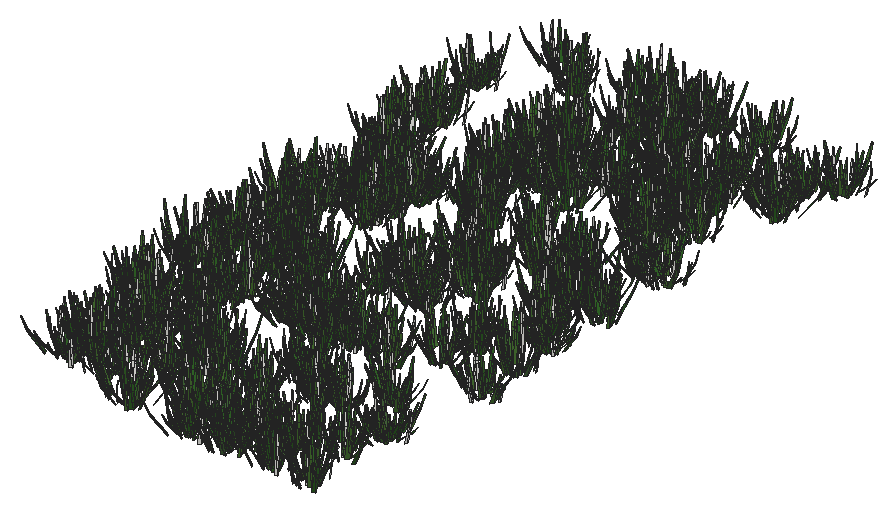
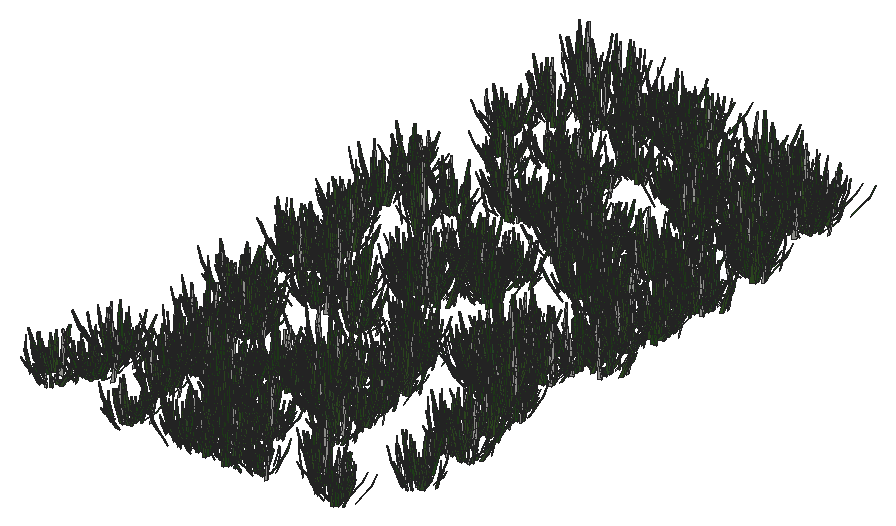
# SketchUp Ruby script. Lengths in inches.
U = 1.inch
M = Sketchup.active_model
def pt(a) = Geom::Point3d.new(a.map { |v| v * U })
def face(e, loops, mat)
  f = e.add_face(loops[0].map { |a| pt(a) })
  loops[1..].each { |l| e.add_face(l.map { |a| pt(a) }).erase! }
  f.material = f.back_material = mat if mat
  f
end
# faces: each face lists its corners as indices into pts; further lists are holes
def faces(e, pts, list, mat = nil) = list.each { |f| face(e, (f[0].is_a?(Array) ? f : [f]).map { |l| l.map { |i| pts[i] } }, mat) }
# xy, xz, yz: faces in a plane at the given z, y or x. An outline is a flat list of corners, or four numbers for a rectangle; further outlines are holes
def ring(l) = l.size == 4 ? [[l[0], l[1]], [l[2], l[1]], [l[2], l[3]], [l[0], l[3]]] : l.each_slice(2).to_a
def flat(e, list, mat, &to3) = list.each { |f| face(e, (f[0].is_a?(Array) ? f : [f]).map { |l| ring(l).map { |u, v| to3.(u, v) } }, mat) }
def xy(e, z, list, mat = nil) = flat(e, list, mat) { |x, y| [x, y, z] }
def xz(e, y, list, mat = nil) = flat(e, list, mat) { |x, z| [x, y, z] }
def yz(e, x, list, mat = nil) = flat(e, list, mat) { |y, z| [x, y, z] }
def lines(e, pts, list) = list.each { |a, b| e.add_line(pt(pts[a]), pt(pts[b])) }
# prism: a flat outline (further loops are holes) pulled along v
def prism(e, loops, v, mat = nil)
  f = face(e, loops, mat); d = Geom::Vector3d.new(v.map { |x| x * U })
  f.pushpull(f.normal.samedirection?(d) ? d.length : -d.length)
end
def box(e, o, s, mat = nil) = prism(e, [[o, [o[0] + s[0], o[1], o[2]], [o[0] + s[0], o[1] + s[1], o[2]], [o[0], o[1] + s[1], o[2]]]], [0, 0, s[2]], mat)
def at(x, y, z, deg = 0) = Geom::Transformation.translation(pt([x, y, z])) * Geom::Transformation.rotation(ORIGIN, Z_AXIS, deg.degrees)
def axes(o, x, y, z) = Geom::Transformation.new([*x, 0, *y, 0, *z, 0, *pt(o).to_a, 1])
def part(name) = M.definitions.add(name)
# library, detail: a bought-in or finely detailed component or shape, given as its bounding box
def library(name, o, s) = part(name).tap { |d| box(d.entities, o, s) }
def detail(e, o, s) = box(e.add_group.entities, o, s)
def put(e, d, t, mat = nil) = e.add_instance(d, t).tap { |i| i.material = mat if mat }
def group(e, t, mat = nil) = e.add_group.tap { |g| g.transformation = t; g.material = mat if mat }.entities
root = M.entities
M.materials.add("Material1").color = [58, 110, 58]
M.materials.add("Material10").color = [48, 100, 38]
M.materials.add("Material3").color = [68, 110, 58]
M.materials.add("Material4").color = [48, 90, 38]
M.materials.add("Material5").color = [68, 110, 48]
M.materials.add("Material6").color = [48, 90, 48]
M.materials.add("Material8").color = [58, 90, 38]
M.materials.add("Material9").color = [68, 100, 58]
c1 = part("grass00")
p = [[-0.6875,0.15,0],[-0.56,0.08,5.52],[-0.04,0.03,2.76],[0.48,-0.02,0],[0.35,-0.02,5.52],[-0.1,-0.14,5.52],
  [-0.12,0.65,8.37],[-0.42,0.65,8.37]]
faces(c1.entities,p,[[0,1,2,3],[3,2,4],[1,5,2],[5,4,2],[1,6,5],[4,5,6],[7,6,1]])
c2 = part("Group16\#1")
put(c2.entities,c1,axes([1.44,-0.61,-0.01],[0.05352,0.12609,0],[-0.10704,0.04543,0.07239],[0.06664,-0.02828,0.11628]),"Material6")
put(c2.entities,c1,axes([0.76,-0.15,-0.01],[0.04676,0.24062,0],[-0.23162,0.04501,0.06642],[0.0652,-0.01267,0.23595]),"Material3")
put(c2.entities,c1,axes([0.79,0.01,-0.01],[-0.00606,0.34651,0],[-0.34381,-0.00602,0.0432],[0.04319,0.00076,0.34386]))
put(c2.entities,c1,axes([1,0.23,-0.01],[-0.07192,0.31144,0],[-0.28722,-0.06632,0.1236],[0.12043,0.02781,0.29478]),"Material5")
put(c2.entities,c1,axes([1.66,0.77,-0.01],[-0.13828,0.29651,0],[-0.21551,-0.1005,0.22471],[0.20365,0.09498,0.23779]),"Material10")
put(c2.entities,c1,axes([0.6875,0.52,-0.01],[-0.18126,0.24051,0],[-0.22746,-0.17142,0.09788],[0.07817,0.05891,0.28481]),"Material5")
put(c2.entities,c1,axes([0.68,0.78,-0.01],[-0.215,0.18688,0],[-0.12385,-0.14248,0.21334],[0.13995,0.16101,0.18878]),"Material3")
put(c2.entities,c1,axes([0.56,1,-0.01],[-0.13756,0.07624,0],[-0.06159,-0.11112,0.0927],[0.04494,0.08108,0.12705]),"Material5")
put(c2.entities,c1,axes([0.2,0.64,-0.01],[-0.23729,0.07254,0],[-0.05711,-0.18681,0.153],[0.04473,0.14632,0.19535]),"Material10")
put(c2.entities,c1,axes([0.0625,0.72,-0.01],[-0.28874,0.02525,0],[-0.02179,-0.24916,0.14647],[0.01276,0.14591,0.25012]),"Material3")
put(c2.entities,c1,axes([-0.08,0.62,-0.01],[-0.34089,-0.04187,0],[0.03255,-0.26504,0.216],[-0.02633,0.21439,0.26703]),"Material10")
put(c2.entities,c1,axes([-0.34,0.98,-0.01],[-0.14314,-0.0493,0],[0.04397,-0.12769,0.06843],[-0.02228,0.0647,0.13505]),"Material10")
put(c2.entities,c1,axes([-0.87,1.45,-0.01],[-0.23488,-0.14114,0],[0.13761,-0.22901,0.06087],[-0.03135,0.05217,0.26717]))
put(c2.entities,c1,axes([-0.72,0.77,-0.01],[-0.14208,-0.13251,0],[0.07209,-0.0773,0.16301],[-0.11118,0.11922,0.1057]),"Material10")
put(c2.entities,c1,axes([-0.62,0.43,-0.01],[-0.14845,-0.21203,0],[0.18654,-0.13061,0.12304],[-0.10079,0.07057,0.22772]),"Material3")
put(c2.entities,c1,axes([-0.68,0.29,-0.01],[-0.13639,-0.32136,0],[0.31723,-0.13464,0.05579],[-0.05136,0.0218,0.34462]),"Material4")
put(c2.entities,c1,axes([-0.64,0.125,-0.01],[-0.0458,-0.23569,0],[0.22124,-0.043,0.08276],[-0.08124,0.01579,0.22538]),"Material1")
put(c2.entities,c1,axes([-1.6,-0.03,-0.01],[0.00576,-0.32897,0],[0.27526,0.00482,0.18018],[-0.18015,-0.00315,0.2753]),"Material5")
put(c2.entities,c1,axes([-1.36,-0.31,-0.01],[0.05718,-0.24765,0],[0.18172,0.04196,0.17267],[-0.16825,-0.03885,0.1865]),"Material10")
put(c2.entities,c1,axes([-1.54,-0.72,-0.01],[0.06537,-0.14017,0],[0.13555,0.06321,0.03939],[-0.0357,-0.01665,0.14956]))
put(c2.entities,c1,axes([-1.19,-0.9,-0.01],[0.09597,-0.12735,0],[0.11214,0.08451,0.07557],[-0.06035,-0.04548,0.14042]),"Material9")
put(c2.entities,c1,axes([-0.47,-0.54,-0.01],[0.11588,-0.10072,0],[0.0618,0.0711,0.12124],[-0.07953,-0.0915,0.0942]))
put(c2.entities,c1,axes([-0.47,-0.84,-0.01],[0.11927,-0.0661,0],[0.06603,0.11913,0.00646],[-0.00313,-0.00565,0.13621]),"Material5")
put(c2.entities,c1,axes([-0.38,-1.24,-0.01],[0.28037,-0.08571,0],[0.0618,0.20215,0.20315],[-0.05939,-0.19428,0.21139]),"Material9")
put(c2.entities,c1,axes([-0.06,-0.66,-0.01],[0.22719,-0.01987,0],[0.01247,0.14255,0.17758],[-0.01547,-0.17691,0.1431]),"Material8")
put(c2.entities,c1,axes([0.11,-0.89,-0.01],[0.14882,0.01828,0],[-0.01058,0.08611,0.12229],[0.01491,-0.12138,0.08676]),"Material6")
put(c2.entities,c1,axes([0.25,-0.72,-0.01],[0.20481,0.07053,0],[-0.06206,0.18022,0.10291],[0.03351,-0.0973,0.1906]),"Material6")
put(c2.entities,c1,axes([0.85,-1.42,-0.01],[0.16481,0.09904,0],[-0.09472,0.15762,0.05616],[0.02893,-0.04814,0.18389]),"Material5")
put(c2.entities,c1,axes([1.01,-1.09,-0.01],[0.21858,0.20385,0],[-0.17495,0.1876,0.15339],[0.10462,-0.11218,0.25652]),"Material10")
put(c2.entities,c1,axes([1.01,-0.71,-0.01],[0.08733,0.12473,0],[-0.06445,0.04512,0.13037],[0.1068,-0.07477,0.07867]),"Material6")
c3 = part("Group15\#1")
put(c3.entities,c2,at(0,0,0))
c4 = part("3darcstudiotree_grass00\#1")
put(c4.entities,c3,at(0,0,0))
put(root,c4,axes([266.63,149.92,0.25],[0.11832,-0.90209,0],[1.15181,0.10407,-0.01362],[0.0181,0.00164,1.54899]))
put(root,c4,axes([266.78,156.0625,0.25],[-0.41827,-0.82788,0],[0.89307,-0.31084,-0.00949],[0.01479,-0.00515,1.63563]))
put(root,c4,axes([266.66,132.55,0.25],[1.08145,-0.17396,0],[0.22673,0.97104,-0.01483],[0.00358,0.01533,1.51152]))
put(root,c4,axes([266.69,119.58,0.25],[0.9093,-0.11168,0],[0.17815,0.99924,-0.00326],[0.00074,0.00416,1.88794]))
put(root,c4,axes([267.35,124.625,0.25],[0.29688,-0.84514,0],[0.95389,0.23084,-0.01207],[0.0194,0.00469,1.66287]))
put(root,c4,axes([267.53,113.35,0.25],[0.74966,-0.72506,0],[0.97919,0.69745,-0.00643],[0.0064,0.00456,1.6911]))
put(root,c4,axes([267.34,125.71,0.25],[-0.10595,0.91113,0],[-1.28961,-0.10331,-0.01578],[-0.01661,-0.00133,1.37044]))
put(root,c4,axes([267.95,128.55,0.25],[0.0172,-0.77777,0],[0.95911,0.01461,-0.01436],[0.02357,0.00036,1.57494]))
put(root,c4,axes([267.98,121.14,0.25],[-0.95988,0.19926,0],[-0.23912,-0.79356,-0.00789],[-0.00334,-0.0111,1.7222]))
put(root,c4,axes([268.02,142.66,0.25],[0.4695,-0.70663,0],[1.00497,0.46,-0.00061],[0.0009,0.00041,1.94394]))
put(root,c4,axes([267.85,146.125,0.25],[-0.53703,0.81953,0],[-1.05808,-0.47764,-0.01158],[-0.01249,-0.00564,1.47884]))
put(root,c4,axes([268.24,149.69,0.25],[-0.12977,-1.05454,0],[1.04338,-0.08845,-0.01024],[0.01776,-0.00151,1.82793]))
put(root,c4,axes([268.14,120.0625,0.25],[0.73343,-0.81835,0],[1.02996,0.63591,-0.01386],[0.01131,0.00698,1.30579]))
put(root,c4,axes([267.84,112.04,0.25],[0.14567,0.90163,0],[-1.1911,0.13257,-0.0098],[-0.01393,0.00155,1.72283]))
put(root,c4,axes([268.28,104.87,0.25],[0.42351,0.77812,0],[-0.98412,0.36899,-0.01637],[-0.01899,0.00712,1.37485]))
put(root,c4,axes([269,102.05,0.25],[-1.20428,-0.04852,0],[0.06041,-1.03281,-0.01036],[0.00056,-0.00964,1.39846]))
put(root,c4,axes([268.94,128.83,0.25],[-0.90448,0.59722,0],[-0.77928,-0.81305,-0.00639],[-0.00513,-0.00535,1.6128]))
put(root,c4,axes([268.92,133.57,0.25],[1.15556,-0.0935,0],[0.12179,1.03693,-0.00515],[0.00072,0.00613,1.80879]))
put(root,c4,axes([269.5,131.83,0.25],[-1.13958,-0.08696,0],[0.09994,-0.90217,-0.01686],[0.00195,-0.01765,1.38194]))
put(root,c4,axes([269.05,110.47,0.25],[0.7679,0.45354,0],[-0.62885,0.73349,-0.00585],[-0.00528,0.00615,1.68777]))
put(root,c4,axes([269.44,103.68,0.25],[0.2797,-0.81879,0],[0.88491,0.20825,-0.01712],[0.02526,0.00594,1.41054]))
put(root,c4,axes([269.5625,136.33,0.25],[0.25817,-0.81695,0],[1.04148,0.22674,-0.01105],[0.01513,0.00329,1.52421]))
put(root,c4,axes([269.3,142.09,0.25],[-0.02064,0.97179,0],[-1.21511,-0.01778,-0.00958],[-0.01169,-0.00017,1.48335]))
put(root,c4,axes([269.78,105.84,0.25],[1.09348,0.34706,0],[-0.42654,0.9258,-0.01506],[-0.00689,0.01496,1.52965]))
put(root,c4,axes([270.31,102.99,0.25],[0.52311,-0.78581,0],[0.8042,0.36881,-0.00396],[0.00733,0.00336,1.94458]))
put(root,c4,axes([270.33,104.8,0.25],[-1.08419,0.52179,0],[-0.50393,-0.72133,-0.01457],[-0.00973,-0.01393,1.33777]))
put(root,c4,axes([270.46,162.01,0.25],[-1.03678,0.10829,0],[-0.12019,-0.79266,-0.01354],[-0.00249,-0.01641,1.41676]))
put(root,c4,axes([270.78,109.26,0.25],[-0.29283,-0.81566,0],[1.20027,-0.29686,-0.01047],[0.01413,-0.0035,1.7643]))
put(root,c4,axes([270.63,141.92,0.25],[-1.16407,0.36188,0],[-0.32044,-0.71009,-0.01358],[-0.0077,-0.01707,1.47772]))
put(root,c4,axes([270.85,115.63,0.25],[-0.80407,-0.34346,0],[0.58115,-0.93725,-0.00712],[0.00423,-0.00682,1.64666]))
put(root,c4,axes([270.72,110.59,0.25],[-0.517,0.73856,0],[-1.06516,-0.51365,-0.00809],[-0.01087,-0.00524,1.91363]))
put(root,c4,axes([270.83,107.38,0.25],[0.87647,-0.17552,0],[0.25218,0.86752,-0.01591],[0.00459,0.01579,1.32206]))
put(root,c4,axes([271.19,124.5,0.25],[0.20033,-0.98018,0],[1.22934,0.17309,-0.00997],[0.0117,0.00165,1.48373]))
put(root,c4,axes([271.16,137.48,0.25],[-0.9323,-0.04265,0],[0.06191,-0.93232,-0.00601],[0.00053,-0.00794,1.79325]))
put(root,c4,axes([270.85,105.56,0.25],[1.12034,0.05805,0],[-0.07391,0.98273,-0.00965],[-0.0008,0.01059,1.57035]))
put(root,c4,axes([271.95,108.4,0.25],[-1.16541,0.21263,0],[-0.22255,-0.8403,-0.01858],[-0.00517,-0.01952,1.34303]))
put(root,c4,axes([272.03,140.58,0.25],[0.71077,0.82893,0],[-0.78621,0.46442,-0.01154],[-0.01284,0.00759,1.31865]))
put(root,c4,axes([272.64,123.17,0.25],[-0.10652,-0.75163,0],[0.99707,-0.09734,-0.01277],[0.01746,-0.0017,1.38207]))
put(root,c4,axes([272.45,101.87,0.25],[-0.44693,0.94214,0],[-0.95359,-0.31163,-0.00571],[-0.00945,-0.00309,1.8245]))
put(root,c4,axes([272.75,116.25,0.25],[0.76834,0.52239,0],[-0.57753,0.58519,-0.00694],[-0.00769,0.00779,1.5947]))
put(root,c4,axes([273.27,126,0.25],[-0.87085,-0.23542,0],[0.37072,-0.94471,-0.00123],[0.00062,-0.00159,1.95221]))
put(root,c4,axes([273.38,160.07,0.25],[0.23595,-0.77044,0],[0.93183,0.19659,-0.00558],[0.00943,0.00199,1.6757]))
put(root,c4,axes([273.3,118.41,0.25],[0.89276,-0.53448,0],[0.66179,0.76152,-0.00659],[0.00667,0.00767,1.95827]))
put(root,c4,axes([273.54,133.32,0.25],[0.95063,-0.17685,0],[0.20528,0.76015,-0.01015],[0.00366,0.01354,1.54623]))
put(root,c4,axes([273.53,134.48,0.25],[-0.34589,0.796,0],[-0.96979,-0.29031,-0.00809],[-0.0133,-0.00398,1.80065]))
put(root,c4,axes([273.71,138.32,0.25],[0.80532,-0.52249,0],[0.73694,0.7825,-0.00613],[0.00551,0.00586,1.74641]))
put(root,c4,axes([273.77,136,0.25],[-0.76955,0.58727,0],[-0.79916,-0.72141,-0.0061],[-0.00641,-0.00579,1.83281]))
put(root,c4,axes([274.12,102.93,0.25],[-1.08191,0.0072,0],[-0.00944,-0.97751,-0.00779],[-0.00009,-0.00939,1.71052]))
put(root,c4,axes([275,139.46,0.25],[-0.21814,-0.94508,0],[0.92117,-0.14647,-0.01579],[0.02401,-0.00382,1.45182]))
put(root,c4,axes([275.09,123.14,0.25],[1.034,0.16058,0],[-0.18896,0.83821,-0.00485],[-0.00152,0.00676,1.75633]))
put(root,c4,axes([275.39,110.7,0.25],[0.38116,0.72172,0],[-1.03898,0.37801,-0.01361],[-0.0176,0.0064,1.60179]))
put(root,c4,axes([275.71,124.43,0.25],[0.76995,0.77633,0],[-0.77001,0.5261,-0.01155],[-0.01518,0.01037,1.69697]))
put(root,c4,axes([276.32,108.76,0.25],[-0.87281,-0.23175,0],[0.37866,-0.98242,-0.00535],[0.0022,-0.00572,1.67969]))
put(root,c4,axes([276.51,154.47,0.25],[-0.22414,-0.83679,0],[1.04153,-0.19219,-0.01455],[0.01817,-0.00335,1.36448]))
put(root,c4,axes([276.54,109.1875,0.25],[-0.5915,0.82087,0],[-0.82708,-0.41056,-0.01081],[-0.01328,-0.00659,1.38013]))
put(root,c4,axes([276.46,151.08,0.25],[-0.06374,0.81035,0],[-1.035,-0.05608,-0.01044],[-0.01512,-0.00082,1.50484]))
put(root,c4,axes([277.21,145.09,0.25],[-0.30384,-0.75904,0],[0.90136,-0.24856,-0.00285],[0.00551,-0.00152,1.93438]))
put(root,c4,axes([277.27,147.72,0.25],[-1.0547,-0.11618,0],[0.16088,-1.00614,-0.01228],[0.00216,-0.01353,1.63767]))
put(root,c4,axes([277.14,104.62,0.25],[-0.80753,0.44806,0],[-0.50831,-0.63112,-0.00767],[-0.00762,-0.00947,1.63569]))
put(root,c4,axes([277.03,99.35,0.25],[1.14358,-0.02006,0],[0.02704,1.06185,-0.00824],[0.00022,0.00855,1.59977]))
put(root,c4,axes([278.24,107.37,0.25],[-0.98679,-0.13086,0],[0.16562,-0.86037,-0.01241],[0.00246,-0.01276,1.31731]))
put(root,c4,axes([278.5,117.46,0.25],[-0.43073,-0.8852,0],[1.04189,-0.34926,-0.01424],[0.01686,-0.00565,1.43479]))
put(root,c4,axes([277.99,162.14,0.25],[0.80627,0.34851,0],[-0.55999,0.89248,-0.0178],[-0.00887,0.01414,1.30843]))
put(root,c4,axes([278.67,119.16,0.25],[-0.95041,-0.18696,0],[0.29853,-1.04549,-0.00987],[0.00261,-0.00914,1.48448]))
put(root,c4,axes([278.28,144.36,0.25],[-0.07869,0.75757,0],[-1.21082,-0.08664,-0.00545],[-0.00867,-0.00062,1.93955]))
put(root,c4,axes([278.87,140.77,0.25],[-1.05804,-0.04604,0],[0.0488,-0.77259,-0.00586],[0.00056,-0.00893,1.71352]))
put(root,c4,axes([279.41,117.57,0.25],[-1.01248,-0.64403,0],[0.7338,-0.79472,-0.01589],[0.01112,-0.01204,1.38765]))
put(root,c4,axes([279.32,108.23,0.25],[0.82484,0.55847,0],[-0.62001,0.63085,-0.0073],[-0.00912,0.00928,1.93831]))
put(root,c4,axes([279.53,152.02,0.25],[1.04481,-0.0802,0],[0.10218,0.91704,-0.00914],[0.00145,0.01297,1.90465]))
put(root,c4,axes([280.36,139.36,0.25],[0.5474,-0.60496,0],[0.84401,0.52611,-0.00267],[0.00378,0.00236,1.87177]))
put(root,c4,axes([280.35,151.4,0.25],[0.01821,0.86082,0],[-1.26514,0.01844,-0.00579],[-0.00839,0.00012,1.83497]))
put(root,c4,axes([281.09,125.55,0.25],[-0.70783,-0.49263,0],[0.7679,-0.7601,-0.0116],[0.00874,-0.00866,1.40225]))
put(root,c4,axes([280.8125,120.53,0.25],[0.87459,-0.34348,0],[0.40101,0.70342,-0.01286],[0.00857,0.01503,1.45976]))
put(root,c4,axes([281.18,157.83,0.25],[-0.28439,-0.91573,0],[1.09091,-0.2334,-0.01269],[0.01847,-0.00395,1.69312]))
put(root,c4,axes([281.12,162.27,0.25],[-1.17771,0.34385,0],[-0.30225,-0.71316,-0.00518],[-0.00352,-0.0083,1.86492]))
put(root,c4,axes([281.03,146.23,0.25],[-0.81557,0.79392,0],[-0.76182,-0.53913,-0.01811],[-0.0179,-0.01267,1.30017]))
put(root,c4,axes([281.28,129.6,0.25],[-1.16841,-0.13889,0],[0.16247,-0.94156,-0.00988],[0.00216,-0.01252,1.76639]))
put(root,c4,axes([281.36,101.73,0.25],[0.38152,-0.99539,0],[1.19985,0.31682,-0.00448],[0.00607,0.0016,1.79011]))
put(root,c4,axes([281.39,117.37,0.25],[-0.91572,-0.09059,0],[0.13318,-0.92744,-0.01308],[0.00226,-0.01576,1.64432]))
put(root,c4,axes([281.39,156.43,0.25],[0.5914,-0.90502,0],[0.93869,0.42257,-0.01711],[0.02021,0.0091,1.43496]))
put(root,c4,axes([281.1,139.4375,0.25],[0.88655,0.24546,0],[-0.34896,0.86829,-0.00681],[-0.00373,0.00927,1.90695]))
put(root,c4,axes([281.6,148.7,0.25],[0.03341,-0.99122,0],[1.18921,0.02761,-0.00421],[0.00642,0.00015,1.81536]))
put(root,c4,axes([281.42,119.51,0.25],[0.88128,0.69098,0],[-0.88475,0.77737,-0.01632],[-0.01273,0.01119,1.46423]))
put(root,c4,axes([282.51,128.38,0.25],[0.3879,-0.82658,0],[1.02977,0.33292,-0.0174],[0.01911,0.00618,1.30214]))
put(root,c4,axes([282.64,102.15,0.25],[0.15714,-0.97551,0],[1.20953,0.13422,-0.0102],[0.01465,0.00163,1.76846]))
put(root,c4,axes([282.79,127.13,0.25],[-1.02045,0.46729,0],[-0.50636,-0.76177,-0.01481],[-0.0098,-0.01474,1.43556]))
put(root,c4,axes([282.82,159.54,0.25],[0.75845,-0.64398,0],[0.7651,0.62077,-0.00015],[0.00019,0.00016,1.98495]))
put(root,c4,axes([283.14,116.13,0.25],[-0.60448,-0.9094,0],[1.03493,-0.4739,-0.0117],[0.01486,-0.0068,1.7149]))
put(root,c4,axes([283.92,162.24,0.25],[-1.0925,-0.23551,0],[0.29257,-0.93497,-0.00758],[0.00281,-0.00899,1.7185]))
put(root,c4,axes([284.25,98.07,0.25],[-1.06215,-0.39029,0],[0.39106,-0.73317,-0.0129],[0.00713,-0.01338,1.31952]))
put(root,c4,axes([284.38,126.86,0.25],[-0.47789,-0.83016,0],[1.08376,-0.42979,-0.00689],[0.00902,-0.00358,1.74288]))
put(root,c4,axes([284.375,106.79,0.25],[0.63804,-0.66337,0],[0.72718,0.48182,-0.01018],[0.01294,0.00858,1.51436]))
put(root,c4,axes([284.26,145.84,0.25],[1.19808,-0.34992,0],[0.35964,0.84828,-0.0057],[0.00298,0.00704,1.70987]))
put(root,c4,axes([284.72,117.05,0.25],[-0.90027,-0.42575,0],[0.47807,-0.69641,-0.01205],[0.00823,-0.01199,1.33255]))
put(root,c4,axes([284.48,131.97,0.25],[1.1724,-0.38255,0],[0.36223,0.76475,-0.00849],[0.00564,0.01192,1.79934]))
put(root,c4,axes([284.83,149.8,0.25],[-1.03664,0.02129,0],[-0.03066,-1.02825,-0.01248],[-0.00034,-0.01147,1.37214]))
put(root,c4,axes([284.71,101.58,0.25],[1.12542,0.30028,0],[-0.30825,0.79588,-0.00634],[-0.00335,0.00866,1.74238]))
put(root,c4,axes([285.6,133.2,0.25],[-1.05845,0.32986,0],[-0.36868,-0.81498,-0.01194],[-0.00686,-0.01516,1.71307]))
put(root,c4,axes([285.39,110.89,0.25],[0.56354,0.75855,0],[-0.83017,0.42488,-0.00763],[-0.01055,0.0054,1.58363]))
put(root,c4,axes([285.96,156.42,0.25],[-0.84155,-0.79069,0],[0.70462,-0.51663,-0.00245],[0.00369,-0.0027,1.8862]))
put(root,c4,axes([285.99,125.57,0.25],[-0.91289,-0.13618,0],[0.19362,-0.89418,-0.01818],[0.00397,-0.01835,1.35222]))
put(root,c4,axes([285.95,149.86,0.25],[-1.06597,0.35425,0],[-0.41198,-0.85402,-0.00598],[-0.00341,-0.00707,1.70205]))
put(root,c4,axes([285.57,117.41,0.25],[1.15133,0.40151,0],[-0.40569,0.8014,-0.00848],[-0.006,0.01186,1.91304]))
put(root,c4,axes([285.67,162.03,0.25],[0.73489,0.5654,0],[-0.84351,0.75529,-0.0132],[-0.01148,0.01028,1.58767]))
put(root,c4,axes([286.23,139.53,0.25],[0.45286,0.76248,0],[-1.10091,0.45044,-0.01549],[-0.01609,0.00658,1.42146]))
put(root,c4,axes([286.98,131.84,0.25],[-0.54754,-0.69769,0],[0.99916,-0.54019,-0.00487],[0.00598,-0.00323,1.74651]))
put(root,c4,axes([287.22,154.47,0.25],[-1.17271,0.05802,0],[-0.06963,-0.96954,-0.00226],[-0.00022,-0.003,1.87745]))
put(root,c4,axes([287.08,110.37,0.25],[0.61057,-0.62706,0],[0.7667,0.51429,-0.01488],[0.01596,0.01071,1.35946]))
put(root,c4,axes([287.15,129.72,0.25],[-0.95062,0.70419,0],[-0.8251,-0.76732,-0.01139],[-0.01081,-0.01006,1.76647]))
put(root,c4,axes([287.51,153.51,0.25],[0.57804,-0.6799,0],[0.85639,0.50158,-0.01427],[0.01458,0.00854,1.30992]))
put(root,c4,axes([287.7,98.24,0.25],[0.82812,0.56873,0],[-0.77872,0.78113,-0.00662],[-0.00566,0.00568,1.63949]))
put(root,c4,axes([288.4,102.48,0.25],[-0.75022,-0.47241,0],[0.57076,-0.62443,-0.01586],[0.01545,-0.0169,1.52204]))
put(root,c4,axes([288.58,117.53,0.25],[0.63417,-0.84147,0],[1.01022,0.52449,-0.01393],[0.01433,0.00744,1.44657]))
put(root,c4,axes([288.46,108.625,0.25],[-0.50673,0.68651,0],[-0.79574,-0.40463,-0.01687],[-0.02097,-0.01067,1.36079]))
put(root,c4,axes([288.65,99.73,0.25],[0.26938,0.92418,0],[-1.18073,0.23709,-0.01063],[-0.01265,0.00254,1.48723]))
put(root,c4,axes([289.25,152.71,0.25],[0.2641,-1.04815,0],[0.90946,0.15787,-0.01603],[0.02507,0.00435,1.48463]))
put(root,c4,axes([288.98,136.42,0.25],[-0.23568,1.05795,0],[-1.26218,-0.1937,-0.00297],[-0.0043,-0.00066,1.8915]))
put(root,c4,axes([290.71,109.41,0.25],[-0.16059,0.73684,0],[-0.93926,-0.14102,-0.01415],[-0.02092,-0.00314,1.43376]))
put(root,c4,axes([290.85,152.48,0.25],[-0.53973,0.62691,0],[-0.91276,-0.54136,-0.01309],[-0.01489,-0.00883,1.56859]))
put(root,c4,axes([290.9,162.22,0.25],[0.35374,0.98258,0],[-0.87439,0.21686,-0.01522],[-0.0222,0.00551,1.38916]))
put(root,c4,axes([291.02,138.66,0.25],[1.1134,0.43982,0],[-0.42198,0.73591,-0.01473],[-0.00962,0.01678,1.49308]))
put(root,c4,axes([292.04,102.08,0.25],[-0.14242,-0.84871,0],[0.98867,-0.11429,-0.01078],[0.01924,-0.00222,1.79898]))
put(root,c4,axes([292.05,135.03,0.25],[0.33889,-0.91019,0],[0.8716,0.22356,-0.00928],[0.01824,0.00468,1.87692]))
put(root,c4,axes([292,120.05,0.25],[0.95759,-0.67869,0],[0.64113,0.62318,-0.01134],[0.01125,0.01093,1.5074]))
put(root,c4,axes([292.01,157.08,0.25],[0.43748,0.73145,0],[-0.95296,0.39264,-0.01001],[-0.0124,0.00511,1.4706]))
put(root,c4,axes([292.54,98.03,0.25],[-0.93614,-0.18607,0],[0.22141,-0.76739,-0.00326],[0.00155,-0.00536,1.93944]))
put(root,c4,axes([292.15,145.76,0.25],[0.85898,0.60765,0],[-0.62831,0.61187,-0.00613],[-0.00688,0.0067,1.67562]))
put(root,c4,axes([292.32,144.87,0.25],[0.4239,0.87591,0],[-1.1209,0.3737,-0.00669],[-0.00997,0.00332,1.94122]))
put(root,c4,axes([293.13,154.64,0.25],[-1.00965,-0.13974,0],[0.15319,-0.76247,-0.01602],[0.00399,-0.01988,1.41148]))
put(root,c4,axes([293.16,122.99,0.25],[0.45748,-1.00116,0],[0.85001,0.26758,-0.00605],[0.01216,0.00383,1.95327]))
put(root,c4,axes([293.39,148.53,0.25],[-1.244,0.10415,0],[-0.09842,-0.8098,-0.00469],[-0.00094,-0.00774,1.96044]))
put(root,c4,axes([293.42,112.11,0.25],[-0.79712,0.74944,0],[-0.78566,-0.57568,-0.01581],[-0.01505,-0.01103,1.33135]))
put(root,c4,axes([293.21,152.28,0.25],[1.10447,0.17095,0],[-0.20618,0.91767,-0.00417],[-0.00127,0.00567,1.87295]))
put(root,c4,axes([293.92,143.33,0.25],[0.17494,0.79206,0],[-1.17023,0.17806,-0.00804],[-0.01181,0.0018,1.77733]))
put(root,c4,axes([294.68,133.29,0.25],[-0.28131,-0.80416,0],[0.93737,-0.2259,-0.00444],[0.00815,-0.00196,1.86591]))
put(root,c4,axes([295.26,129.51,0.25],[-0.97164,0.6705,0],[-0.69811,-0.69693,-0.00935],[-0.00886,-0.00884,1.61847]))
put(root,c4,axes([295.48,103.39,0.25],[0.75831,-0.87609,0],[0.78153,0.46602,-0.0087],[0.0118,0.00703,1.60603]))
put(root,c4,axes([295.45,147.71,0.25],[0.35623,0.77552,0],[-0.9578,0.30309,-0.01397],[-0.01938,0.00613,1.52193]))
put(root,c4,axes([296.19,140.13,0.25],[-0.98027,-0.22948,0],[0.26234,-0.77201,-0.015],[0.00551,-0.0162,1.30652]))
put(root,c4,axes([296.16,134.72,0.25],[-0.85384,0.78104,0],[-0.79795,-0.60095,-0.0082],[-0.00975,-0.00734,1.73071]))
put(root,c4,axes([296.28,98.17,0.25],[0.44737,-0.94973,0],[0.88957,0.28867,-0.00888],[0.01622,0.00526,1.87213]))
put(root,c4,axes([296.47,127.39,0.25],[-0.26229,-0.88232,0],[0.94327,-0.19317,-0.01268],[0.02035,-0.00417,1.60602]))
put(root,c4,axes([296.68,107.34,0.25],[-0.54407,-0.91228,0],[0.86118,-0.35382,-0.01272],[0.0163,-0.0067,1.37453]))
put(root,c4,axes([297.48,126.84,0.25],[-0.29225,0.82352,0],[-1.06145,-0.25949,-0.01201],[-0.01521,-0.00372,1.46096]))
put(root,c4,axes([297.58,155.7,0.25],[0.41008,0.74842,0],[-0.90906,0.34314,-0.00419],[-0.00662,0.0025,1.73548]))
put(root,c4,axes([297.64,122.23,0.25],[0.03706,0.78393,0],[-1.13415,0.03693,-0.00595],[-0.01038,0.00034,1.98232]))
put(root,c4,axes([297.68,132.64,0.25],[0.88218,0.47435,0],[-0.5947,0.76194,-0.01048],[-0.0081,0.01038,1.55517]))
put(root,c4,axes([297.68,158.35,0.25],[0.72727,0.83743,0],[-0.84781,0.50723,-0.01552],[-0.01735,0.01038,1.43977]))
put(root,c4,axes([298.17,117.375,0.25],[-0.96742,0.39922,0],[-0.4877,-0.81417,-0.01143],[-0.00629,-0.01049,1.35283]))
put(root,c4,axes([297.93,154.64,0.25],[1.17388,-0.06991,0],[0.09013,1.04254,-0.01186],[0.00103,0.01187,1.52253]))
put(root,c4,axes([297.89,140.61,0.25],[0.36751,0.93998,0],[-1.10245,0.29694,-0.01715],[-0.01987,0.00535,1.41194]))
put(root,c4,axes([299.87,160.81,0.25],[-0.25082,-0.89805,0],[1.22427,-0.23556,-0.01344],[0.01489,-0.00287,1.42931]))
